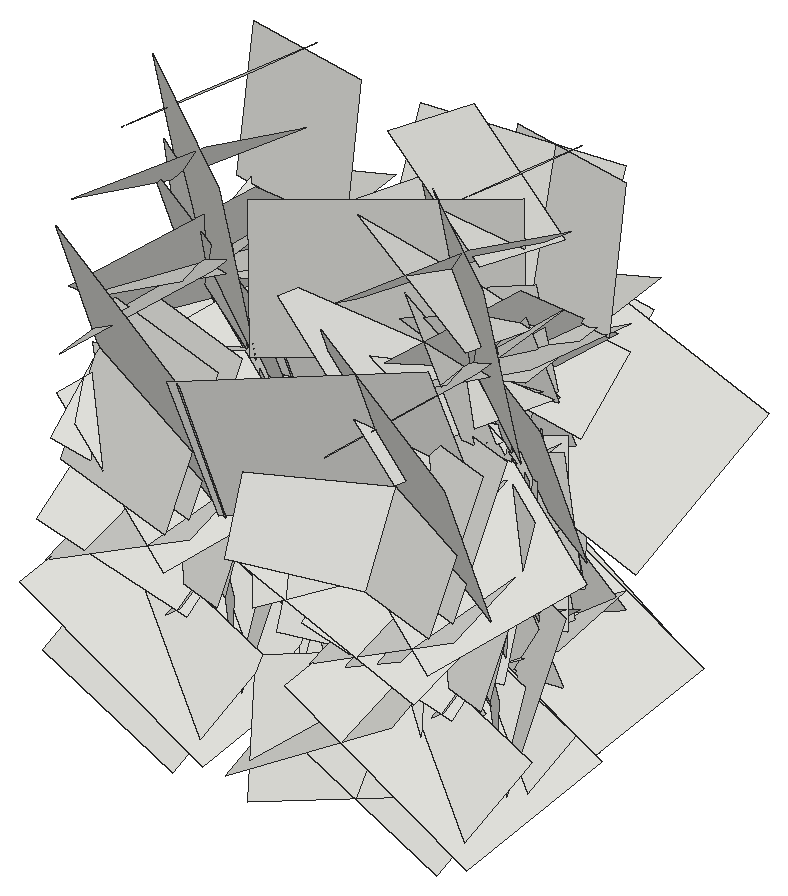
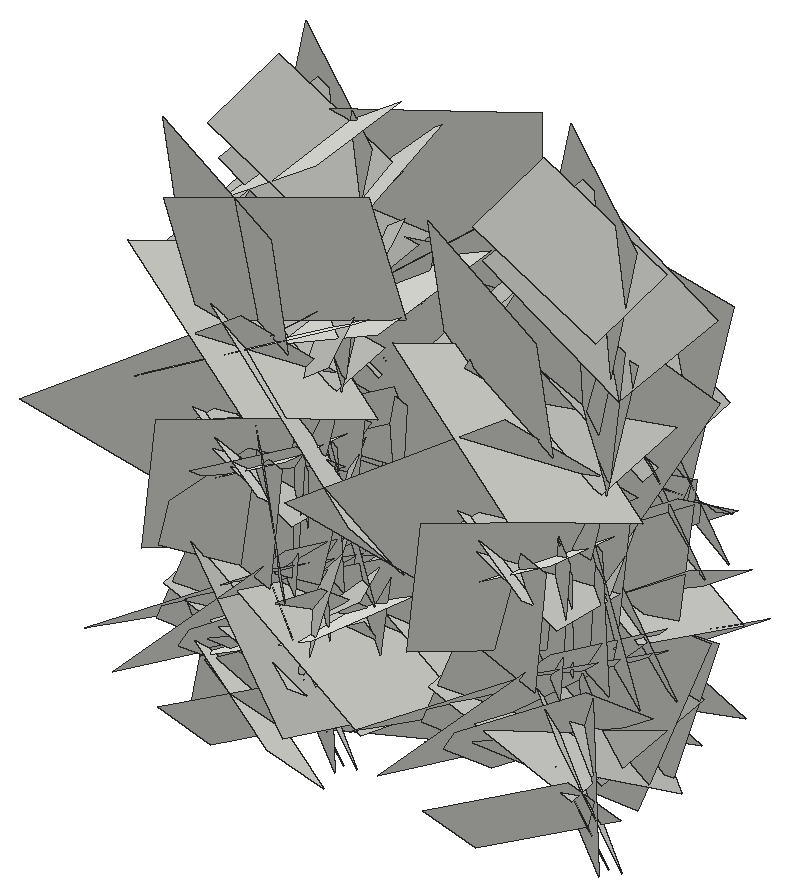
# SketchUp Ruby script. Lengths in inches.
U = 1.inch
M = Sketchup.active_model
def pt(a) = Geom::Point3d.new(a.map { |v| v * U })
def face(e, loops, mat)
  f = e.add_face(loops[0].map { |a| pt(a) })
  loops[1..].each { |l| e.add_face(l.map { |a| pt(a) }).erase! }
  f.material = f.back_material = mat if mat
  f
end
# faces: each face lists its corners as indices into pts; further lists are holes
def faces(e, pts, list, mat = nil) = list.each { |f| face(e, (f[0].is_a?(Array) ? f : [f]).map { |l| l.map { |i| pts[i] } }, mat) }
# xy, xz, yz: faces in a plane at the given z, y or x. An outline is a flat list of corners, or four numbers for a rectangle; further outlines are holes
def ring(l) = l.size == 4 ? [[l[0], l[1]], [l[2], l[1]], [l[2], l[3]], [l[0], l[3]]] : l.each_slice(2).to_a
def flat(e, list, mat, &to3) = list.each { |f| face(e, (f[0].is_a?(Array) ? f : [f]).map { |l| ring(l).map { |u, v| to3.(u, v) } }, mat) }
def xy(e, z, list, mat = nil) = flat(e, list, mat) { |x, y| [x, y, z] }
def xz(e, y, list, mat = nil) = flat(e, list, mat) { |x, z| [x, y, z] }
def yz(e, x, list, mat = nil) = flat(e, list, mat) { |y, z| [x, y, z] }
def lines(e, pts, list) = list.each { |a, b| e.add_line(pt(pts[a]), pt(pts[b])) }
# prism: a flat outline (further loops are holes) pulled along v
def prism(e, loops, v, mat = nil)
  f = face(e, loops, mat); d = Geom::Vector3d.new(v.map { |x| x * U })
  f.pushpull(f.normal.samedirection?(d) ? d.length : -d.length)
end
def box(e, o, s, mat = nil) = prism(e, [[o, [o[0] + s[0], o[1], o[2]], [o[0] + s[0], o[1] + s[1], o[2]], [o[0], o[1] + s[1], o[2]]]], [0, 0, s[2]], mat)
def at(x, y, z, deg = 0) = Geom::Transformation.translation(pt([x, y, z])) * Geom::Transformation.rotation(ORIGIN, Z_AXIS, deg.degrees)
def axes(o, x, y, z) = Geom::Transformation.new([*x, 0, *y, 0, *z, 0, *pt(o).to_a, 1])
def part(name) = M.definitions.add(name)
# library, detail: a bought-in or finely detailed component or shape, given as its bounding box
def library(name, o, s) = part(name).tap { |d| box(d.entities, o, s) }
def detail(e, o, s) = box(e.add_group.entities, o, s)
def put(e, d, t, mat = nil) = e.add_instance(d, t).tap { |i| i.material = mat if mat }
def group(e, t, mat = nil) = e.add_group.tap { |g| g.transformation = t; g.material = mat if mat }.entities
root = M.entities
c1 = part("Component\#6")
p = [[0.01,0,0],[0,3.24,4.54],[4.32,3.24,4.54],[4.33,0,0]]
faces(c1.entities,p,[[0,1,2,3]])
put(root,c1,axes([24.34,124,36.29],[-0.02149,0.52903,-1.24729],[0.2007,-1.23408,-0.5265],[1.42204,0.18216,0.05546]))
put(root,c1,axes([38.11,124,36.29],[0.02149,0.52903,-1.24729],[-0.2007,-1.23408,-0.5265],[-1.42204,0.18216,0.05546]))
put(root,c1,axes([34.14,124,36.29],[-0.02149,0.52903,-1.24729],[0.2007,-1.23408,-0.5265],[1.42204,0.18216,0.05546]))
put(root,c1,axes([24.28,123.49,22.43],[0.36857,0.54861,0.76203],[0.54406,0.56941,-0.64413],[0.83345,-0.61431,0.08349]))
put(root,c1,axes([38.17,123.49,22.43],[-0.36857,0.54861,0.76203],[-0.54406,0.56941,-0.64413],[-0.83345,-0.61431,0.08349]))
put(root,c1,axes([34.09,123.49,22.43],[0.36857,0.54861,0.76203],[0.54406,0.56941,-0.64413],[0.83345,-0.61431,0.08349]))
put(root,c1,axes([24.34,126.73,32.74],[-0.07983,-0.47542,-1.06148],[0.1788,-1.05692,0.46141],[1.21984,0.1238,-0.1371]))
put(root,c1,axes([38.11,126.73,32.74],[0.07983,-0.47542,-1.06148],[-0.1788,-1.05692,0.46141],[-1.21984,0.1238,-0.1371]))
put(root,c1,axes([34.14,126.73,32.74],[-0.07983,-0.47542,-1.06148],[0.1788,-1.05692,0.46141],[1.21984,0.1238,-0.1371]))
put(root,c1,axes([24.34,122.33,25.2],[0.14417,1.26196,0.33106],[0.05821,0.32703,-1.26913],[1.38172,-0.14545,0.01892]))
put(root,c1,axes([38.11,122.33,25.2],[-0.14417,1.26196,0.33106],[-0.05821,0.32703,-1.26913],[-1.38172,-0.14545,0.01892]))
put(root,c1,axes([34.14,122.33,25.2],[0.14417,1.26196,0.33106],[0.05821,0.32703,-1.26913],[1.38172,-0.14545,0.01892]))
put(root,c1,axes([24.34,127.85,32.74],[-0.07983,-0.47542,-1.06148],[0.1788,-1.05692,0.46141],[1.21984,0.1238,-0.1371]))
put(root,c1,axes([38.11,127.85,32.74],[0.07983,-0.47542,-1.06148],[-0.1788,-1.05692,0.46141],[-1.21984,0.1238,-0.1371]))
put(root,c1,axes([34.14,127.85,32.74],[-0.07983,-0.47542,-1.06148],[0.1788,-1.05692,0.46141],[1.21984,0.1238,-0.1371]))
put(root,c1,axes([24.34,128.39,27.01],[0.01413,-1.13969,-0.35832],[0.11214,-0.35581,1.13564],[1.2614,0.04439,-0.09695]))
put(root,c1,axes([34.14,128.39,27.01],[0.01413,-1.13969,-0.35832],[0.11214,-0.35581,1.13564],[1.2614,0.04439,-0.09695]))
put(root,c1,axes([38.11,128.39,27.01],[-0.01413,-1.13969,-0.35832],[-0.11214,-0.35581,1.13564],[-1.2614,0.04439,-0.09695]))
put(root,c1,axes([23.63,124.93,30.08],[0.69154,0.83647,0.57299],[0.50453,0.34895,-1.05134],[0.94895,-0.79509,0.14141]))
put(root,c1,axes([38.83,124.93,30.08],[-0.69154,0.83647,0.57299],[-0.50453,0.34895,-1.05134],[-0.94895,-0.79509,0.14141]))
put(root,c1,axes([33.43,124.93,30.08],[0.69154,0.83647,0.57299],[0.50453,0.34895,-1.05134],[0.94895,-0.79509,0.14141]))
put(root,c1,axes([34.14,128.06,26.23],[-0.10092,-0.80547,-0.37503],[-0.00485,-0.37672,0.81027],[0.94179,-0.08825,-0.03602]))
put(root,c1,axes([28.31,128.06,26.23],[0.10092,-0.80547,-0.37503],[0.00485,-0.37672,0.81027],[-0.94179,-0.08825,-0.03602]))
put(root,c1,axes([38.11,128.06,26.23],[0.10092,-0.80547,-0.37503],[0.00485,-0.37672,0.81027],[-0.94179,-0.08825,-0.03602]))
put(root,c1,axes([24.34,128.2,32.33],[0.15852,-1.12421,0.05612],[-0.12401,0.04078,1.12872],[1.18668,0.15444,0.11046]))
put(root,c1,axes([38.11,128.2,32.33],[-0.15852,-1.12421,0.05612],[0.12401,0.04078,1.12872],[-1.18668,0.15444,0.11046]))
put(root,c1,axes([34.14,128.2,32.33],[0.15852,-1.12421,0.05612],[-0.12401,0.04078,1.12872],[1.18668,0.15444,0.11046]))
put(root,c1,axes([24.28,125.55,22.43],[0.36857,0.54861,0.76203],[0.54406,0.56941,-0.64413],[0.83345,-0.61431,0.08349]))
put(root,c1,axes([38.17,125.55,22.43],[-0.36857,0.54861,0.76203],[-0.54406,0.56941,-0.64413],[-0.83345,-0.61431,0.08349]))
put(root,c1,axes([34.09,125.55,22.43],[0.36857,0.54861,0.76203],[0.54406,0.56941,-0.64413],[0.83345,-0.61431,0.08349]))
put(root,c1,axes([34.14,129.13,29.07],[-0.11411,-0.79222,-0.47459],[-0.01099,-0.47673,0.79815],[0.97884,-0.0977,-0.04636]))
put(root,c1,axes([28.31,129.13,29.07],[0.11411,-0.79222,-0.47459],[0.01099,-0.47673,0.79815],[-0.97884,-0.0977,-0.04636]))
put(root,c1,axes([38.11,129.13,29.07],[0.11411,-0.79222,-0.47459],[0.01099,-0.47673,0.79815],[-0.97884,-0.0977,-0.04636]))
put(root,c1,axes([24.34,128.47,40.0625],[0.15368,0.21217,-1.35934],[-0.08132,-1.3635,-0.221],[1.45608,-0.09854,0.13113]))
put(root,c1,axes([34.14,128.47,40.0625],[0.15368,0.21217,-1.35934],[-0.08132,-1.3635,-0.221],[1.45608,-0.09854,0.13113]))
put(root,c1,axes([38.11,128.47,40.0625],[-0.15368,0.21217,-1.35934],[0.08132,-1.3635,-0.221],[-1.45608,-0.09854,0.13113]))
put(root,c1,axes([24.34,129.14,29.25],[-0.07983,-0.47542,-1.06148],[0.1788,-1.05692,0.46141],[1.21984,0.1238,-0.1371]))
put(root,c1,axes([34.14,129.14,29.25],[-0.07983,-0.47542,-1.06148],[0.1788,-1.05692,0.46141],[1.21984,0.1238,-0.1371]))
put(root,c1,axes([38.11,129.14,29.25],[0.07983,-0.47542,-1.06148],[-0.1788,-1.05692,0.46141],[-1.21984,0.1238,-0.1371]))
put(root,c1,axes([24.34,126.77,21.87],[-0.10992,-0.34124,0.92241],[0.05569,0.92428,0.34784],[1.04103,-0.08548,0.07879]))
put(root,c1,axes([38.11,126.77,21.87],[0.10992,-0.34124,0.92241],[-0.05569,0.92428,0.34784],[-1.04103,-0.08548,0.07879]))
put(root,c1,axes([34.14,126.77,21.87],[-0.10992,-0.34124,0.92241],[0.05569,0.92428,0.34784],[1.04103,-0.08548,0.07879]))
put(root,c1,axes([24.34,129.34,35.47],[-0.09463,-0.94647,0.23979],[-0.00571,0.24126,0.95028],[1.03494,-0.08521,0.02717]))
put(root,c1,axes([34.14,129.34,35.47],[-0.09463,-0.94647,0.23979],[-0.00571,0.24126,0.95028],[1.03494,-0.08521,0.02717]))
put(root,c1,axes([38.11,129.34,35.47],[0.09463,-0.94647,0.23979],[0.00571,0.24126,0.95028],[-1.03494,-0.08521,0.02717]))
put(root,c1,axes([24.34,130.61,23.63],[-0.04049,-0.92661,-0.53015],[-0.18829,-0.51758,0.91743],[1.11583,-0.12096,0.13557]))
put(root,c1,axes([34.14,130.61,23.63],[-0.04049,-0.92661,-0.53015],[-0.18829,-0.51758,0.91743],[1.11583,-0.12096,0.13557]))
put(root,c1,axes([38.11,130.61,23.63],[0.04049,-0.92661,-0.53015],[0.18829,-0.51758,0.91743],[-1.11583,-0.12096,0.13557]))
put(root,c1,axes([24.34,126.5625,26.98],[-0.04661,-0.13743,1.04442],[0.16266,1.03335,0.14244],[1.10472,-0.15795,0.02309]))
put(root,c1,axes([38.11,126.5625,26.98],[0.04661,-0.13743,1.04442],[-0.16266,1.03335,0.14244],[-1.10472,-0.15795,0.02309]))
put(root,c1,axes([34.14,126.5625,26.98],[-0.04661,-0.13743,1.04442],[0.16266,1.03335,0.14244],[1.10472,-0.15795,0.02309]))
put(root,c1,axes([34.14,128.14,26.625],[-0.13018,-0.67547,0.62862],[-0.07474,0.63918,0.67304],[0.97523,-0.04118,0.13549]))
put(root,c1,axes([28.31,128.14,26.625],[0.13018,-0.67547,0.62862],[0.07474,0.63918,0.67304],[-0.97523,-0.04118,0.13549]))
put(root,c1,axes([38.11,128.14,26.625],[0.13018,-0.67547,0.62862],[0.07474,0.63918,0.67304],[-0.97523,-0.04118,0.13549]))
put(root,c1,axes([24.34,130.48,31.34],[-0.20009,-0.24055,-1.32848],[-0.01815,-1.34087,0.24522],[1.43098,-0.05064,-0.18264]))
put(root,c1,axes([34.14,130.48,31.34],[-0.20009,-0.24055,-1.32848],[-0.01815,-1.34087,0.24522],[1.43098,-0.05064,-0.18264]))
put(root,c1,axes([38.11,130.48,31.34],[0.20009,-0.24055,-1.32848],[0.01815,-1.34087,0.24522],[-1.43098,-0.05064,-0.18264]))
put(root,c1,axes([28.31,126.29,27.49],[0.18614,0.86586,-0.34095],[0.04817,-0.35453,-0.87695],[-0.98523,0.14625,-0.10729]))
put(root,c1,axes([34.14,126.29,27.49],[-0.18614,0.86586,-0.34095],[-0.04817,-0.35453,-0.87695],[0.98523,0.14625,-0.10729]))
put(root,c1,axes([38.11,126.29,27.49],[0.18614,0.86586,-0.34095],[0.04817,-0.35453,-0.87695],[-0.98523,0.14625,-0.10729]))
put(root,c1,axes([24.34,130.13,32.75],[0.05656,-1.14018,0.16245],[0.17438,0.16851,1.12862],[1.20828,0.02906,-0.17049]))
put(root,c1,axes([34.14,130.13,32.75],[0.05656,-1.14018,0.16245],[0.17438,0.16851,1.12862],[1.20828,0.02906,-0.17049]))
put(root,c1,axes([38.11,130.13,32.75],[-0.05656,-1.14018,0.16245],[-0.17438,0.16851,1.12862],[-1.20828,0.02906,-0.17049]))
put(root,c1,axes([24.34,128.45,36.29],[-0.02149,0.52903,-1.24729],[0.2007,-1.23408,-0.5265],[1.42204,0.18216,0.05546]))
put(root,c1,axes([38.11,128.45,36.29],[0.02149,0.52903,-1.24729],[-0.2007,-1.23408,-0.5265],[-1.42204,0.18216,0.05546]))
put(root,c1,axes([34.14,128.45,36.29],[-0.02149,0.52903,-1.24729],[0.2007,-1.23408,-0.5265],[1.42204,0.18216,0.05546]))
put(root,c1,axes([24.34,129.02,36.97],[-0.03047,0.19902,-0.90037],[0.05941,-0.89877,-0.20045],[0.97562,0.06094,-0.01591]))
put(root,c1,axes([34.14,129.02,36.97],[-0.03047,0.19902,-0.90037],[0.05941,-0.89877,-0.20045],[0.97562,0.06094,-0.01591]))
put(root,c1,axes([38.11,129.02,36.97],[0.03047,0.19902,-0.90037],[-0.05941,-0.89877,-0.20045],[-0.97562,0.06094,-0.01591]))
put(root,c1,axes([24.34,130.54,26.21],[-0.16316,0.13144,-1.2549],[-0.21583,-1.25022,-0.10597],[1.31994,-0.18819,-0.17245]))
put(root,c1,axes([38.11,130.54,26.21],[0.16316,0.13144,-1.2549],[0.21583,-1.25022,-0.10597],[-1.31994,-0.18819,-0.17245]))
put(root,c1,axes([34.14,130.54,26.21],[-0.16316,0.13144,-1.2549],[-0.21583,-1.25022,-0.10597],[1.31994,-0.18819,-0.17245]))
put(root,c1,axes([24.34,129.15,30.625],[-0.089,-0.93417,0.70597],[-0.20388,0.70917,0.91554],[1.22433,0.05019,0.20378]))
put(root,c1,axes([34.14,129.15,30.625],[-0.089,-0.93417,0.70597],[-0.20388,0.70917,0.91554],[1.22433,0.05019,0.20378]))
put(root,c1,axes([38.11,129.15,30.625],[0.089,-0.93417,0.70597],[0.20388,0.70917,0.91554],[-1.22433,0.05019,0.20378]))
put(root,c1,axes([24.34,132.16,25.41],[-0.07094,-0.60211,-1.2376],[-0.1162,-1.23279,0.6057],[1.45423,-0.12788,-0.01197]))
put(root,c1,axes([34.14,132.16,25.41],[-0.07094,-0.60211,-1.2376],[-0.1162,-1.23279,0.6057],[1.45423,-0.12788,-0.01197]))
put(root,c1,axes([38.11,132.16,25.41],[0.07094,-0.60211,-1.2376],[0.1162,-1.23279,0.6057],[-1.45423,-0.12788,-0.01197]))
put(root,c1,axes([24.34,130.09,30.86],[-0.13772,0.10296,-1.023],[-0.01142,-1.03121,-0.10242],[1.08979,0.0022,-0.13035]))
put(root,c1,axes([34.14,130.09,30.86],[-0.13772,0.10296,-1.023],[-0.01142,-1.03121,-0.10242],[1.08979,0.0022,-0.13035]))
put(root,c1,axes([38.11,130.09,30.86],[0.13772,0.10296,-1.023],[0.01142,-1.03121,-0.10242],[-1.08979,0.0022,-0.13035]))
put(root,c1,axes([24.34,130.39,37.85],[0.05885,-0.83818,0.13983],[-0.03078,0.13818,0.83979],[0.90022,0.05952,0.01957]))
put(root,c1,axes([34.14,130.39,37.85],[0.05885,-0.83818,0.13983],[-0.03078,0.13818,0.83979],[0.90022,0.05952,0.01957]))
put(root,c1,axes([38.11,130.39,37.85],[-0.05885,-0.83818,0.13983],[0.03078,0.13818,0.83979],[-0.90022,0.05952,0.01957]))
put(root,c1,axes([24.34,128.44,21.53],[-0.07533,-0.68545,1.00594],[-0.30491,0.98857,0.65329],[1.25377,0.19923,0.21932]))
put(root,c1,axes([34.14,128.44,21.53],[-0.07533,-0.68545,1.00594],[-0.30491,0.98857,0.65329],[1.25377,0.19923,0.21932]))
put(root,c1,axes([38.11,128.44,21.53],[0.07533,-0.68545,1.00594],[0.30491,0.98857,0.65329],[-1.25377,0.19923,0.21932]))
put(root,c1,axes([24.34,131.26,22.93],[0.10206,-0.4663,-0.72841],[0.02316,-0.73136,0.47108],[0.91647,0.07041,0.06921]))
put(root,c1,axes([34.14,131.26,22.93],[0.10206,-0.4663,-0.72841],[0.02316,-0.73136,0.47108],[0.91647,0.07041,0.06921]))
put(root,c1,axes([38.11,131.26,22.93],[-0.10206,-0.4663,-0.72841],[-0.02316,-0.73136,0.47108],[-0.91647,0.07041,0.06921]))
put(root,c1,axes([24.34,131.47,30.67],[0.19347,-0.24403,-0.96391],[-0.05093,-0.98104,0.23927],[1.05275,-0.00261,0.18872]))
put(root,c1,axes([34.14,131.47,30.67],[0.19347,-0.24403,-0.96391],[-0.05093,-0.98104,0.23927],[1.05275,-0.00261,0.18872]))
put(root,c1,axes([38.11,131.47,30.67],[-0.19347,-0.24403,-0.96391],[0.05093,-0.98104,0.23927],[-1.05275,-0.00261,0.18872]))
put(root,c1,axes([24.34,131.58,31.0625],[0.07279,0.01987,-1.05868],[-0.10279,-1.05633,-0.02611],[1.11768,-0.09844,0.06655]))
put(root,c1,axes([34.14,131.58,31.0625],[0.07279,0.01987,-1.05868],[-0.10279,-1.05633,-0.02611],[1.11768,-0.09844,0.06655]))
put(root,c1,axes([38.11,131.58,31.0625],[-0.07279,0.01987,-1.05868],[0.10279,-1.05633,-0.02611],[-1.11768,-0.09844,0.06655]))
put(root,c1,axes([24.34,131.52,23.18],[0.15485,-0.9106,-0.00305],[0.11373,0.01414,0.91588],[0.95852,0.14543,-0.10818]))
put(root,c1,axes([34.14,131.52,23.18],[0.15485,-0.9106,-0.00305],[0.11373,0.01414,0.91588],[0.95852,0.14543,-0.10818]))
put(root,c1,axes([38.11,131.52,23.18],[-0.15485,-0.9106,-0.00305],[-0.11373,0.01414,0.91588],[-0.95852,0.14543,-0.10818]))
put(root,c1,axes([24.34,127.05,26.22],[0.14417,1.26196,0.33106],[0.05821,0.32703,-1.26913],[1.38172,-0.14545,0.01892]))
put(root,c1,axes([38.11,127.05,26.22],[-0.14417,1.26196,0.33106],[-0.05821,0.32703,-1.26913],[-1.38172,-0.14545,0.01892]))
put(root,c1,axes([34.14,127.05,26.22],[0.14417,1.26196,0.33106],[0.05821,0.32703,-1.26913],[1.38172,-0.14545,0.01892]))
put(root,c1,axes([24.34,127.73,24.28],[-0.02979,0.75993,0.53946],[-0.00151,0.53967,-0.7603],[0.98786,0.02374,0.0151]))
put(root,c1,axes([38.11,127.73,24.28],[0.02979,0.75993,0.53946],[0.00151,0.53967,-0.7603],[-0.98786,0.02374,0.0151]))
put(root,c1,axes([34.14,127.73,24.28],[-0.02979,0.75993,0.53946],[-0.00151,0.53967,-0.7603],[0.98786,0.02374,0.0151]))
put(root,c1,axes([24.34,127.1,26.99],[-0.01407,1.25738,0.35681],[-0.29384,0.346,-1.2296],[1.35392,0.08816,-0.26315]))
put(root,c1,axes([38.11,127.1,26.99],[0.01407,1.25738,0.35681],[0.29384,0.346,-1.2296],[-1.35392,0.08816,-0.26315]))
put(root,c1,axes([34.14,127.1,26.99],[-0.01407,1.25738,0.35681],[-0.29384,0.346,-1.2296],[1.35392,0.08816,-0.26315]))
put(root,c1,axes([24.34,129.03,31.05],[0.04043,0.74356,0.04678],[0.07255,0.04314,-0.74161],[0.78639,-0.04221,0.06601]))
put(root,c1,axes([34.14,129.03,31.05],[0.04043,0.74356,0.04678],[0.07255,0.04314,-0.74161],[0.78639,-0.04221,0.06601]))
put(root,c1,axes([28.31,129.03,31.05],[-0.04043,0.74356,0.04678],[-0.07255,0.04314,-0.74161],[-0.78639,-0.04221,0.06601]))
put(root,c1,axes([38.11,129.03,31.05],[-0.04043,0.74356,0.04678],[-0.07255,0.04314,-0.74161],[-0.78639,-0.04221,0.06601]))
put(root,c1,axes([24.34,134.48,33.76],[-0.26334,-1.11466,-0.41014],[0.1173,-0.43892,1.12584],[1.25351,-0.19309,-0.19152]))
put(root,c1,axes([38.11,134.48,33.76],[0.26334,-1.11466,-0.41014],[-0.1173,-0.43892,1.12584],[-1.25351,-0.19309,-0.19152]))
put(root,c1,axes([34.14,134.48,33.76],[-0.26334,-1.11466,-0.41014],[0.1173,-0.43892,1.12584],[1.25351,-0.19309,-0.19152]))
put(root,c1,axes([28.31,133.52,31.89],[0.15087,-0.04242,-1.05475],[0.23169,-1.04005,0.07132],[-1.09469,-0.22597,-0.13027]))
put(root,c1,axes([34.14,133.52,31.89],[-0.15087,-0.04242,-1.05475],[-0.23169,-1.04005,0.07132],[1.09469,-0.22597,-0.13027]))
put(root,c1,axes([38.11,133.52,31.89],[0.15087,-0.04242,-1.05475],[0.23169,-1.04005,0.07132],[-1.09469,-0.22597,-0.13027]))
put(root,c1,axes([24.34,129.22,21.54],[-0.01805,0.58513,0.55019],[0.06792,0.54955,-0.58247],[0.84865,-0.03153,0.05832]))
put(root,c1,axes([34.14,129.22,21.54],[-0.01805,0.58513,0.55019],[0.06792,0.54955,-0.58247],[0.84865,-0.03153,0.05832]))
put(root,c1,axes([38.11,129.22,21.54],[0.01805,0.58513,0.55019],[-0.06792,0.54955,-0.58247],[-0.84865,-0.03153,0.05832]))
put(root,c1,axes([34.14,129.75,30.06],[0.01937,0.49926,0.36665],[0.0577,0.36409,-0.4985],[0.65405,-0.04691,0.03312]))
put(root,c1,axes([28.31,129.75,30.06],[-0.01937,0.49926,0.36665],[-0.0577,0.36409,-0.4985],[-0.65405,-0.04691,0.03312]))
put(root,c1,axes([38.11,129.75,30.06],[-0.01937,0.49926,0.36665],[-0.0577,0.36409,-0.4985],[-0.65405,-0.04691,0.03312]))
put(root,c1,axes([24.34,133.17,39.1],[0.0845,-0.28698,-1.03421],[0.22383,-1.0126,0.29726],[1.11545,0.22493,0.0187]))
put(root,c1,axes([38.11,133.17,39.1],[-0.0845,-0.28698,-1.03421],[-0.22383,-1.0126,0.29726],[-1.11545,0.22493,0.0187]))
put(root,c1,axes([34.14,133.17,39.1],[0.0845,-0.28698,-1.03421],[0.22383,-1.0126,0.29726],[1.11545,0.22493,0.0187]))
put(root,c1,axes([24.34,128.43,31.91],[0.33386,1.00192,0.91989],[0.02581,0.93993,-1.03208],[1.44154,-0.24887,-0.19457]))
put(root,c1,axes([34.14,128.43,31.91],[0.33386,1.00192,0.91989],[0.02581,0.93993,-1.03208],[1.44154,-0.24887,-0.19457]))
put(root,c1,axes([38.11,128.43,31.91],[-0.33386,1.00192,0.91989],[-0.02581,0.93993,-1.03208],[-1.44154,-0.24887,-0.19457]))
put(root,c1,axes([34.14,130.92,26.67],[-0.06799,-0.20959,0.7931],[0.02884,0.79454,0.21217],[0.86907,-0.04277,0.05501]))
put(root,c1,axes([28.31,130.92,26.67],[0.06799,-0.20959,0.7931],[-0.02884,0.79454,0.21217],[-0.86907,-0.04277,0.05501]))
put(root,c1,axes([38.11,130.92,26.67],[0.06799,-0.20959,0.7931],[-0.02884,0.79454,0.21217],[-0.86907,-0.04277,0.05501]))
